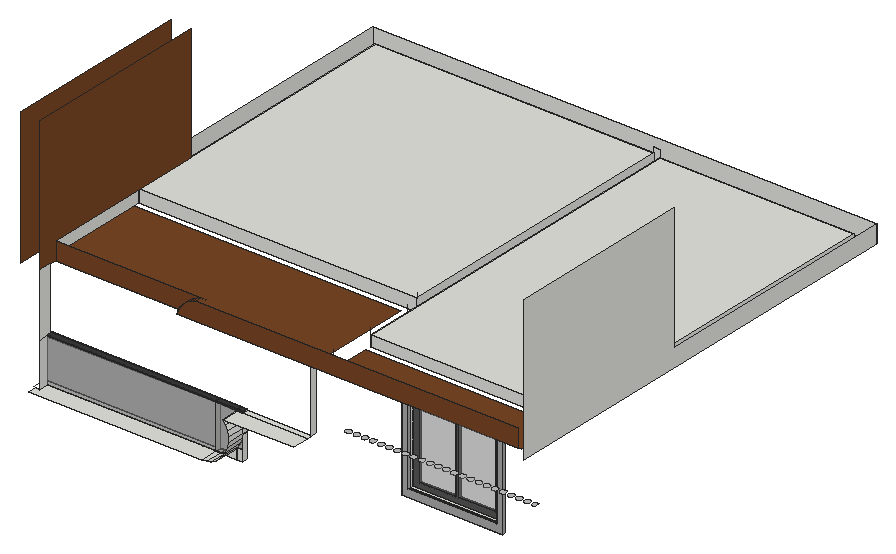
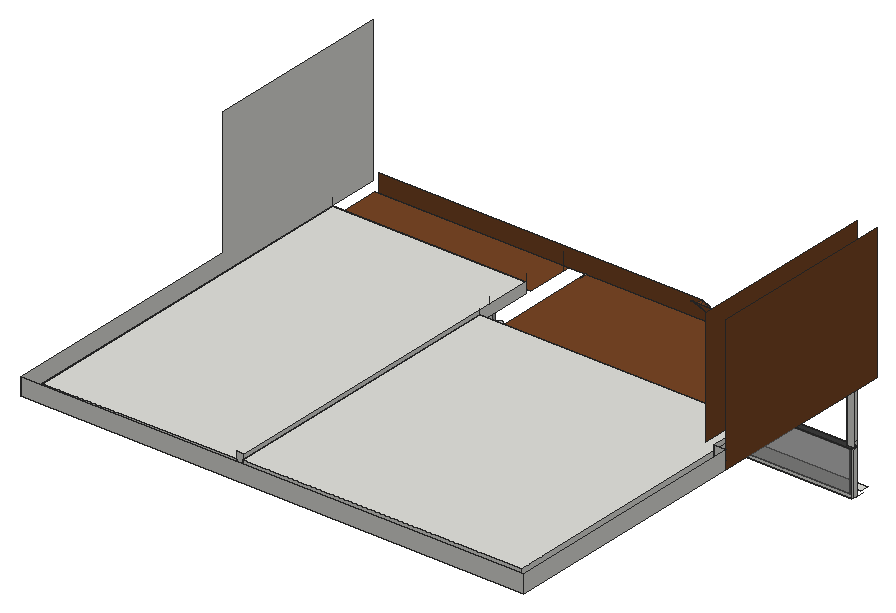
# SketchUp Ruby script. Lengths in millimetres.
U = 1.mm
M = Sketchup.active_model
def pt(a) = Geom::Point3d.new(a.map { |v| v * U })
def face(e, loops, mat)
  f = e.add_face(loops[0].map { |a| pt(a) })
  loops[1..].each { |l| e.add_face(l.map { |a| pt(a) }).erase! }
  f.material = f.back_material = mat if mat
  f
end
# faces: each face lists its corners as indices into pts; further lists are holes
def faces(e, pts, list, mat = nil) = list.each { |f| face(e, (f[0].is_a?(Array) ? f : [f]).map { |l| l.map { |i| pts[i] } }, mat) }
# xy, xz, yz: faces in a plane at the given z, y or x. An outline is a flat list of corners, or four numbers for a rectangle; further outlines are holes
def ring(l) = l.size == 4 ? [[l[0], l[1]], [l[2], l[1]], [l[2], l[3]], [l[0], l[3]]] : l.each_slice(2).to_a
def flat(e, list, mat, &to3) = list.each { |f| face(e, (f[0].is_a?(Array) ? f : [f]).map { |l| ring(l).map { |u, v| to3.(u, v) } }, mat) }
def xy(e, z, list, mat = nil) = flat(e, list, mat) { |x, y| [x, y, z] }
def xz(e, y, list, mat = nil) = flat(e, list, mat) { |x, z| [x, y, z] }
def yz(e, x, list, mat = nil) = flat(e, list, mat) { |y, z| [x, y, z] }
def lines(e, pts, list) = list.each { |a, b| e.add_line(pt(pts[a]), pt(pts[b])) }
# prism: a flat outline (further loops are holes) pulled along v
def prism(e, loops, v, mat = nil)
  f = face(e, loops, mat); d = Geom::Vector3d.new(v.map { |x| x * U })
  f.pushpull(f.normal.samedirection?(d) ? d.length : -d.length)
end
def box(e, o, s, mat = nil) = prism(e, [[o, [o[0] + s[0], o[1], o[2]], [o[0] + s[0], o[1] + s[1], o[2]], [o[0], o[1] + s[1], o[2]]]], [0, 0, s[2]], mat)
def at(x, y, z, deg = 0) = Geom::Transformation.translation(pt([x, y, z])) * Geom::Transformation.rotation(ORIGIN, Z_AXIS, deg.degrees)
def axes(o, x, y, z) = Geom::Transformation.new([*x, 0, *y, 0, *z, 0, *pt(o).to_a, 1])
def part(name) = M.definitions.add(name)
# library, detail: a bought-in or finely detailed component or shape, given as its bounding box
def library(name, o, s) = part(name).tap { |d| box(d.entities, o, s) }
def detail(e, o, s) = box(e.add_group.entities, o, s)
def put(e, d, t, mat = nil) = e.add_instance(d, t).tap { |i| i.material = mat if mat }
def group(e, t, mat = nil) = e.add_group.tap { |g| g.transformation = t; g.material = mat if mat }.entities
root = M.entities
M.materials.add("[Color M03]").color = [170, 170, 170]
M.materials.add("[Color M06]").color = [86, 86, 86]
M.materials.add("[Color M07]").color = [58, 58, 58]
M.materials.add("[Metal Corrugated Shiny]").color = [193, 193, 193]
M.materials.add("[Translucent Glass Gray]").color = [128, 128, 128]
M.materials["[Translucent Glass Gray]"].alpha = 0.5
M.materials.add("[Wood Veneer 01]").color = [120, 70, 37]
c1 = part("Group\#1")
xy(c1.entities,0,[[0,0,1355.7,60.3]],"[Color M06]")
xy(c1.entities,100.1,[[100.1,0,655.5,60.3],[696.9,0,1255.7,60.3]],"[Color M06]")
xy(c1.entities,1517.6,[[100.1,0,655.5,60.3],[696.9,0,1255.7,60.3]],"[Color M06]")
xy(c1.entities,1617.7,[[0,0,1355.7,60.3]],"[Color M06]")
xz(c1.entities,0,[[[0,0,1355.7,1617.7],[696.9,100.1,1255.7,1517.6],[100.1,100.1,655.5,1517.6]]],"[Color M06]")
xz(c1.entities,0,[[100.1,100.1,655.5,1517.6],[696.9,100.1,1255.7,1517.6]],"[Translucent Glass Gray]")
xz(c1.entities,60.3,[[[0,0,1355.7,1617.7],[696.9,100.1,1255.7,1517.6],[100.1,100.1,655.5,1517.6]]],"[Color M06]")
yz(c1.entities,0,[[0,0,60.3,1617.7]],"[Color M06]")
yz(c1.entities,100.1,[[0,100.1,60.3,1517.6]],"[Color M06]")
yz(c1.entities,655.5,[[0,100.1,60.3,1517.6]],"[Color M06]")
yz(c1.entities,696.9,[[0,100.1,60.3,1517.6]],"[Color M06]")
yz(c1.entities,1255.7,[[0,100.1,60.3,1517.6]],"[Color M06]")
yz(c1.entities,1355.7,[[0,0,60.3,1617.7]],"[Color M06]")
xy(root,4073.5,[[8130.9,1584.3,10586.8,1657.4]],"[Color M03]")
xy(root,4242.9,[[8275.8,1657.3,10434.8,1809.7]])
xy(root,4242.9,[[8275.8,1584.3,10434.8,1657.3]],"[Color M03]")
xy(root,4272.1,[[374.7,0,4556.2,0,4556.2,424.6,479.5,424.6,479.5,209.6,374.7,209.6],[308.1,424.6,4556.2,555.6],[4556.2,424.6,5081.7,555.6],[5081.7,424.6,5214.2,555.6]])
xy(root,5334,[[5080.9,0,6787.6,424.6],[5080.9,424.6,5081.7,555.6],[5214.2,424.6,6787.6,555.6]])
xy(root,5334,[[308.1,424.6,4556.2,555.6],[4556.2,424.6,5080.9,555.6],[5081.7,424.6,5214.2,555.6]],"[Color M07]")
xy(root,5372.1,[[308.1,424.6,479.5,514.4]])
xy(root,5372.1,[[479.5,424.6,4556.2,424.6,4556.2,555.6,308.1,555.6,308.1,514.4,479.5,514.4],[4556.2,424.6,5080.9,555.6],[5081.7,424.6,5214.2,555.6]],"[Color M07]")
xy(root,5423.4,[[7323,932.9,7339.9,934.9,7355.7,941.2,7369.3,951.3,7379.8,964.7,7386.5,980.3,7389,997.1,7387,1014,7380.7,1029.8,7370.6,1043.4,7357.2,1053.9,7341.6,1060.6,7324.8,1063.1,7307.9,1061.1,7292.1,1054.8,7278.5,1044.7,7268,1031.3,7261.3,1015.7,7258.8,998.9,7260.8,982,7267.1,966.2,7277.2,952.6,7290.6,942.1,7306.2,935.4],[7519.8,932.9,7536.7,934.9,7552.5,941.2,7566.1,951.3,7576.7,964.7,7583.4,980.3,7585.8,997.1,7583.8,1014,7577.6,1029.8,7567.4,1043.4,7554.1,1053.9,7538.5,1060.6,7521.6,1063.1,7504.8,1061.1,7489,1054.8,7475.4,1044.7,7464.8,1031.3,7458.1,1015.7,7455.7,998.9,7457.6,982,7463.9,966.2,7474.1,952.6,7487.4,942.1,7503,935.4],[7716.7,932.9,7733.6,934.9,7749.4,941.2,7763,951.3,7773.5,964.7,7780.2,980.3,7782.7,997.1,7780.7,1014,7774.4,1029.8,7764.3,1043.4,7750.9,1053.9,7735.3,1060.6,7718.5,1063.1,7701.6,1061.1,7685.8,1054.8,7672.2,1044.7,7661.7,1031.3,7655,1015.7,7652.5,998.9,7654.5,982,7660.8,966.2,7670.9,952.6,7684.3,942.1,7699.9,935.4],[7913.5,932.9,7930.4,934.9,7946.2,941.2,7959.8,951.3,7970.4,964.7,7977.1,980.3,7979.5,997.1,7977.5,1014,7971.3,1029.8,7961.1,1043.4,7947.8,1053.9,7932.2,1060.6,7915.3,1063.1,7898.5,1061.1,7882.7,1054.8,7869.1,1044.7,7858.5,1031.3,7851.8,1015.7,7849.4,998.9,7851.3,982,7857.6,966.2,7867.8,952.6,7881.1,942.1,7896.7,935.4],[8110.4,932.9,8127.3,934.9,8143.1,941.2,8156.7,951.3,8167.2,964.7,8173.9,980.3,8176.4,997.1,8174.4,1014,8168.1,1029.8,8158,1043.4,8144.6,1053.9,8129,1060.6,8112.2,1063.1,8095.3,1061.1,8079.5,1054.8,8065.9,1044.7,8055.4,1031.3,8048.7,1015.7,8046.2,998.9,8048.2,982,8054.5,966.2,8064.6,952.6,8078,942.1,8093.6,935.4],
  [8307.2,932.9,8324.1,934.9,8339.9,941.2,8353.5,951.3,8364.1,964.7,8370.8,980.3,8373.2,997.1,8371.2,1014,8365,1029.8,8354.8,1043.4,8341.5,1053.9,8325.9,1060.6,8309,1063.1,8292.2,1061.1,8276.4,1054.8,8262.8,1044.7,8252.2,1031.3,8245.5,1015.7,8243.1,998.9,8245,982,8251.3,966.2,8261.5,952.6,8274.8,942.1,8290.4,935.4],[8504.1,932.9,8521,934.9,8536.8,941.2,8550.4,951.3,8560.9,964.7,8567.6,980.3,8570.1,997.1,8568.1,1014,8561.8,1029.8,8551.7,1043.4,8538.3,1053.9,8522.7,1060.6,8505.9,1063.1,8489,1061.1,8473.2,1054.8,8459.6,1044.7,8449.1,1031.3,8442.4,1015.7,8439.9,998.9,8441.9,982,8448.2,966.2,8458.3,952.6,8471.7,942.1,8487.3,935.4],[8700.9,932.9,8717.8,934.9,8733.6,941.2,8747.2,951.3,8757.8,964.7,8764.5,980.3,8766.9,997.1,8764.9,1014,8758.7,1029.8,8748.5,1043.4,8735.2,1053.9,8719.6,1060.6,8702.7,1063.1,8685.9,1061.1,8670.1,1054.8,8656.5,1044.7,8645.9,1031.3,8639.2,1015.7,8636.8,998.9,8638.7,982,8645,966.2,8655.2,952.6,8668.5,942.1,8684.1,935.4],[8897.8,932.9,8914.7,934.9,8930.5,941.2,8944.1,951.3,8954.6,964.7,8961.3,980.3,8963.8,997.1,8961.8,1014,8955.5,1029.8,8945.4,1043.4,8932,1053.9,8916.4,1060.6,8899.6,1063.1,8882.7,1061.1,8866.9,1054.8,8853.3,1044.7,8842.8,1031.3,8836.1,1015.7,8833.6,998.9,8835.6,982,8841.9,966.2,8852,952.6,8865.4,942.1,8881,935.4],[9094.6,932.9,9111.5,934.9,9127.3,941.2,9140.9,951.3,9151.5,964.7,9158.2,980.3,9160.6,997.1,9158.6,1014,9152.4,1029.8,9142.2,1043.4,9128.9,1053.9,9113.3,1060.6,9096.4,1063.1,9079.6,1061.1,9063.8,1054.8,9050.2,1044.7,9039.6,1031.3,9032.9,1015.7,9030.5,998.9,9032.4,982,9038.7,966.2,9048.9,952.6,9062.2,942.1,9077.8,935.4],
  [9291.5,932.9,9308.4,934.9,9324.2,941.2,9337.8,951.3,9348.3,964.7,9355,980.3,9357.5,997.1,9355.5,1014,9349.2,1029.8,9339.1,1043.4,9325.7,1053.9,9310.1,1060.6,9293.3,1063.1,9276.4,1061.1,9260.6,1054.8,9247,1044.7,9236.5,1031.3,9229.8,1015.7,9227.3,998.9,9229.3,982,9235.6,966.2,9245.7,952.6,9259.1,942.1,9274.7,935.4],[9488.3,932.9,9505.2,934.9,9521,941.2,9534.6,951.3,9545.2,964.7,9551.9,980.3,9554.3,997.1,9552.3,1014,9546.1,1029.8,9535.9,1043.4,9522.6,1053.9,9507,1060.6,9490.1,1063.1,9473.3,1061.1,9457.5,1054.8,9443.9,1044.7,9433.3,1031.3,9426.6,1015.7,9424.2,998.9,9426.1,982,9432.4,966.2,9442.6,952.6,9455.9,942.1,9471.5,935.4],[9685.2,932.9,9702.1,934.9,9717.9,941.2,9731.5,951.3,9742,964.7,9748.7,980.3,9751.2,997.1,9749.2,1014,9742.9,1029.8,9732.8,1043.4,9719.4,1053.9,9703.8,1060.6,9687,1063.1,9670.1,1061.1,9654.3,1054.8,9640.7,1044.7,9630.2,1031.3,9623.5,1015.7,9621,998.9,9623,982,9629.3,966.2,9639.4,952.6,9652.8,942.1,9668.4,935.4],[9882,932.9,9898.9,934.9,9914.7,941.2,9928.3,951.3,9938.9,964.7,9945.6,980.3,9948,997.1,9946,1014,9939.8,1029.8,9929.6,1043.4,9916.3,1053.9,9900.7,1060.6,9883.8,1063.1,9867,1061.1,9851.2,1054.8,9837.6,1044.7,9827,1031.3,9820.3,1015.7,9817.9,998.9,9819.8,982,9826.1,966.2,9836.3,952.6,9849.6,942.1,9865.2,935.4],[10078.9,932.9,10095.8,934.9,10111.6,941.2,10125.2,951.3,10135.7,964.7,10142.4,980.3,10144.9,997.1,10142.9,1014,10136.6,1029.8,10126.5,1043.4,10113.1,1053.9,10097.5,1060.6,10080.7,1063.1,10063.8,1061.1,10048,1054.8,10034.4,1044.7,10023.9,1031.3,10017.2,1015.7,10014.7,998.9,10016.7,982,10023,966.2,10033.1,952.6,10046.5,942.1,10062.1,935.4],
  [10275.7,932.9,10292.6,934.9,10308.4,941.2,10322,951.3,10332.6,964.7,10339.3,980.3,10341.7,997.1,10339.7,1014,10333.5,1029.8,10323.3,1043.4,10310,1053.9,10294.4,1060.6,10277.5,1063.1,10260.7,1061.1,10244.9,1054.8,10231.3,1044.7,10220.7,1031.3,10214,1015.7,10211.6,998.9,10213.5,982,10219.8,966.2,10230,952.6,10243.3,942.1,10258.9,935.4],[10472.6,932.9,10489.5,934.9,10505.3,941.2,10518.9,951.3,10529.4,964.7,10536.1,980.3,10538.6,997.1,10536.6,1014,10530.3,1029.8,10520.2,1043.4,10506.8,1053.9,10491.2,1060.6,10474.4,1063.1,10457.5,1061.1,10441.7,1054.8,10428.1,1044.7,10417.6,1031.3,10410.9,1015.7,10408.4,998.9,10410.4,982,10416.7,966.2,10426.8,952.6,10440.2,942.1,10455.8,935.4],[10669.4,932.9,10686.3,934.9,10702.1,941.2,10715.7,951.3,10726.3,964.7,10733,980.3,10735.4,997.1,10733.4,1014,10727.2,1029.8,10717,1043.4,10703.7,1053.9,10688.1,1060.6,10671.2,1063.1,10654.4,1061.1,10638.6,1054.8,10625,1044.7,10614.4,1031.3,10607.7,1015.7,10605.3,998.9,10607.2,982,10613.5,966.2,10623.7,952.6,10637,942.1,10652.6,935.4],[10866.3,932.9,10883.2,934.9,10899,941.2,10912.6,951.3,10923.1,964.7,10929.8,980.3,10932.3,997.1,10930.3,1014,10924,1029.8,10913.9,1043.4,10900.5,1053.9,10884.9,1060.6,10868.1,1063.1,10851.2,1061.1,10835.4,1054.8,10821.8,1044.7,10811.3,1031.3,10804.6,1015.7,10802.1,998.9,10804.1,982,10810.4,966.2,10820.5,952.6,10833.9,942.1,10849.5,935.4],[11063.1,932.9,11080,934.9,11095.8,941.2,11109.4,951.3,11120,964.7,11126.7,980.3,11129.1,997.1,11127.1,1014,11120.9,1029.8,11110.7,1043.4,11097.4,1053.9,11081.8,1060.6,11064.9,1063.1,11048.1,1061.1,11032.3,1054.8,11018.7,1044.7,11008.1,1031.3,11001.4,1015.7,10999,998.9,11000.9,982,11007.2,966.2,11017.4,952.6,11030.7,942.1,11046.3,935.4],
  [11260,932.9,11276.9,934.9,11292.7,941.2,11306.3,951.3,11316.8,964.7,11323.5,980.3,11326,997.1,11324,1014,11317.7,1029.8,11307.6,1043.4,11294.2,1053.9,11278.6,1060.6,11261.8,1063.1,11244.9,1061.1,11229.1,1054.8,11215.5,1044.7,11205,1031.3,11198.3,1015.7,11195.8,998.9,11197.8,982,11204.1,966.2,11214.2,952.6,11227.6,942.1,11243.2,935.4],[11456.8,932.9,11473.7,934.9,11489.5,941.2,11503.1,951.3,11513.7,964.7,11520.4,980.3,11522.8,997.1,11520.8,1014,11514.6,1029.8,11504.4,1043.4,11491.1,1053.9,11475.5,1060.6,11458.6,1063.1,11441.8,1061.1,11426,1054.8,11412.4,1044.7,11401.8,1031.3,11395.1,1015.7,11392.7,998.9,11394.6,982,11400.9,966.2,11411.1,952.6,11424.4,942.1,11440,935.4],[11653.7,932.9,11670.6,934.9,11686.4,941.2,11700,951.3,11710.5,964.7,11717.2,980.3,11719.7,997.1,11717.7,1014,11711.4,1029.8,11701.3,1043.4,11687.9,1053.9,11672.3,1060.6,11655.5,1063.1,11638.6,1061.1,11622.8,1054.8,11609.2,1044.7,11598.7,1031.3,11592,1015.7,11589.5,998.9,11591.5,982,11597.8,966.2,11607.9,952.6,11621.3,942.1,11636.9,935.4],[11850.5,932.9,11867.4,934.9,11883.2,941.2,11890.5,946.6,11890.5,1049.4,11884.8,1053.9,11869.2,1060.6,11852.3,1063.1,11835.5,1061.1,11819.7,1054.8,11806.1,1044.7,11795.5,1031.3,11788.8,1015.7,11786.4,998.9,11788.3,982,11794.6,966.2,11804.8,952.6,11818.1,942.1,11833.7,935.4]],"[Metal Corrugated Shiny]")
xy(root,6383.1,[[2137.7,3257.5,4426,3410]])
xy(root,6401.9,[[8275.8,1657.3,10434.8,1809.7]])
xy(root,6401.9,[[8275.8,1584.3,10434.8,1657.3]],"[Color M03]")
xy(root,6529.3,[[8130.9,1584.3,10586.8,1657.4]],"[Color M03]")
xy(root,6858,[[308.1,514.4,479.5,687.4]])
xy(root,6858,[[3547.8,514.4,3547.8,687.4,308.1,687.4,308.1,3257.6,6787.6,3257.6,6787.6,514.4],[7199.4,514.4,11890.5,1657.4]],"[Wood Veneer 01]")
xy(root,7112,[[7199.4,1809.8,11890.5,10572.8]])
xy(root,7162.8,[[308.1,3410,7047,10572.8]])
xz(root,424.6,[[308.1,4272.1,479.5,5334],[4556.2,4272.1,5081.7,4272.1,5081.7,4533,5002.2,4445.4,4904.8,4371.6,4795.5,4317,4677.9,4283.4],[5081.7,4272.1,5214.2,4533],[5081.7,4533,5214.2,4533,5214.2,5332.7,5081.7,5332.7,5145.9,5230.5,5190.6,5116.7,5213.7,4996.7,5214.2,4874.4,5192.2,4754.2,5148.4,4640.1,5084.4,4536],[5081.7,5332.7,5081.7,5334,5080.9,5334],
  [5081.7,5332.7,5214.2,5334],[308.1,5334,479.5,5372.1]])
xz(root,424.6,[[479.5,5334,4556.2,5372.1],[4556.2,5334,5080.9,5372.1],[5081.7,5334,5214.2,5372.1]],"[Color M07]")
xz(root,424.6,[[479.5,4272.1,4556.2,5334],[4556.2,4272.1,4677.9,4283.4,4795.5,4317,4904.8,4371.6,5002.2,4445.4,5081.7,4533,5081.7,5332.7,5080.9,5334,4556.2,5334],[5081.7,4533,5214.2,5332.7]],"[Translucent Glass Gray]")
xz(root,514.4,[[308.1,5372.1,479.5,6858]])
xz(root,514.4,[[3547.8,6858,11814.3,6858,11814.3,7289.8,4112.5,7289.8,4048.9,7286.3,3986.1,7276,3924.8,7258.9,3865.8,7235.3,3809.6,7205.3,3757,7169.5,3708.7,7128.1,3665.1,7081.8,3626.8,7031,3594.2,6976.3,3567.8,6918.4]],"[Wood Veneer 01]")
xz(root,555.6,[[4556.2,4272.1,4677.9,4283.4,4795.5,4317,4904.8,4371.6,5002.2,4445.4,5081.7,4533,5081.7,4272.1],[5081.7,4272.1,5214.2,4533],[5081.7,4533,5084.4,4536,5148.4,4640.1,5192.2,4754.2,5214.2,4874.4,5213.7,4996.7,5190.6,5116.7,5145.9,5230.5,5081.7,5332.7,5214.2,5332.7,5214.2,4533],[5081.7,5332.7,5080.9,5334,5081.7,5334],[5081.7,5332.7,5214.2,5334]])
xz(root,555.6,[[308.1,5334,4556.2,5372.1],[4556.2,5334,5080.9,5372.1],[5081.7,5334,5214.2,5372.1]],"[Color M07]")
xz(root,555.6,[[308.1,4272.1,4556.2,5334],[4556.2,4272.1,4556.2,5334,5080.9,5334,5081.7,5332.7,5081.7,4533,5002.2,4445.4,4904.8,4371.6,4795.5,4317,4677.9,4283.4],[5081.7,4533,5214.2,5332.7]],"[Translucent Glass Gray]")
xz(root,687.4,[[308.1,6858,479.5,7289.8]])
xz(root,687.4,[[479.5,6858,3547.8,6858,3567.8,6918.4,3594.2,6976.3,3626.8,7031,3665.1,7081.8,3708.7,7128.1,3757,7169.5,3809.6,7205.3,3865.8,7235.3,3924.8,7258.9,3986.1,7276,4048.9,7286.3,4112.5,7289.8,479.5,7289.8]],"[Wood Veneer 01]")
xz(root,1584.3,[[[8130.9,4073.5,10586.8,6529.3],[8275.8,4242.9,10434.8,6401.9]]],"[Color M03]")
xz(root,1809.8,[[7199.4,6858,11890.5,7112]])
xz(root,3410,[[308.1,6858,7047,7162.8]])
xz(root,4760.9,[[3.3,6858,308.1,7289.8]])
xz(root,10572.8,[[308.1,6858,7047,7162.8],[7047,6858,7199.4,7289.8],[7199.4,6858,11890.5,7112]])
xz(root,10877.6,[[3.3,6858,12195.3,7289.8]])
yz(root,3.3,[[4760.9,6858,10877.6,7289.8]])
yz(root,3.3,[[209.6,6858,4760.9,10119.6]],"[Wood Veneer 01]")
yz(root,308.1,[[424.6,4272.1,514.4,5334],[514.4,4272.1,555.6,5334],[687.4,6858,3410,6858,3410,7162.8,4181.5,7162.8,4181.5,7289.8,687.4,7289.8],[3410,6858,4760.9,7162.8],[4760.9,6858,10572.8,7162.8],
  [4181.5,7162.8,4760.9,7289.8]])
yz(root,308.1,[[424.6,5334,514.4,5372.1],[514.4,5334,555.6,5372.1]],"[Color M07]")
yz(root,479.5,[[209.6,4272.1,424.6,5334],[209.6,5334,424.6,5334,424.6,5372.1,514.4,5372.1,514.4,6858,209.6,6858]])
yz(root,479.5,[[209.6,6858,687.4,6858,687.4,7289.8,4760.9,7289.8,4760.9,10096.5,209.6,10096.5]],"[Wood Veneer 01]")
yz(root,4556.2,[[424.6,4272.1,555.6,5334]])
yz(root,4556.2,[[424.6,5334,555.6,5372.1]],"[Color M07]")
yz(root,5080.9,[[424.6,5334,555.6,5372.1]],"[Color M07]")
yz(root,5081.7,[[424.6,4272.1,555.6,5334]])
yz(root,5081.7,[[424.6,5334,555.6,5372.1]],"[Color M07]")
yz(root,5214.2,[[424.6,4272.1,555.6,4874.4],[424.6,4874.4,555.6,5334]])
yz(root,5214.2,[[424.6,5334,555.6,5372.1]],"[Color M07]")
yz(root,6787.6,[[514.4,5334,687.4,6858]])
yz(root,7047,[[3410,6858,10572.8,7162.8]])
yz(root,7199.4,[[1809.8,6858,10572.8,7112]])
yz(root,8130.9,[[1584.3,4073.5,1657.4,6529.3]],"[Color M03]")
yz(root,8275.8,[[1657.3,4242.9,1809.7,6401.9]])
yz(root,8275.8,[[1584.3,4242.9,1657.3,6401.9]],"[Color M03]")
yz(root,10434.8,[[1657.3,4242.9,1809.7,6401.9]])
yz(root,10434.8,[[1584.3,4242.9,1657.3,6401.9]],"[Color M03]")
yz(root,10586.8,[[1584.3,4073.5,1657.4,6529.3]],"[Color M03]")
yz(root,11890.5,[[1809.8,6858,10572.8,7112]])
yz(root,12195.3,[[209.6,6858,10877.6,6858,10877.6,7289.8,4760.9,7289.8,4760.9,10337.8,209.6,10337.8]])
p = [[8130.9,1657.4,6529.3],[10586.8,1657.4,6529.3],[10586.8,1657.4,4073.5],[8130.9,1657.4,4073.5],[8275.8,1657.3,4242.9],[10434.8,1657.3,4242.9],
  [10434.8,1657.3,6401.9],[8275.8,1657.3,6401.9],[4556.2,424.6,4272.1],[4556.2,0,4272.1],[4677.9,0,4283.4],[4677.9,424.6,4283.4],
  [4677.9,555.6,4283.4],[4556.2,555.6,4272.1],[4795.5,0,4317],[4795.5,424.6,4317],[4795.5,555.6,4317],[4904.8,0,4371.6],
  [4904.8,424.6,4371.6],[4904.8,555.6,4371.6],[5002.2,0,4445.4],[5002.2,424.6,4445.4],[5002.2,555.6,4445.4],[5084.4,0,4536],
  [5084.4,424.6,4536],[5081.7,424.6,4533],[5084.4,555.6,4536],[5081.7,555.6,4533],[5148.4,0,4640.1],[5148.4,424.6,4640.1],
  [5148.4,555.6,4640.1],[5192.2,0,4754.2],[5192.2,424.6,4754.2],[5192.2,555.6,4754.2],[5214.2,0,4874.4],[5214.2,424.6,4874.4],
  [5214.2,555.6,4874.4],[5213.7,0,4996.7],[5213.7,424.6,4996.7],[5213.7,555.6,4996.7],[5190.6,0,5116.7],[5190.6,424.6,5116.7],
  [5190.6,555.6,5116.7],[5145.9,0,5230.5],[5145.9,424.6,5230.5],[5145.9,555.6,5230.5],[5080.9,0,5334],[5080.9,424.6,5334],
  [5081.7,424.6,5332.7],[5080.9,555.6,5334],[5081.7,555.6,5332.7],[3567.8,687.4,6918.4],[3547.8,687.4,6858],[3547.8,514.4,6858],
  [3567.8,514.4,6918.4],[3594.2,687.4,6976.3],[3594.2,514.4,6976.3],[3626.8,687.4,7031],[3626.8,514.4,7031],[3665.1,687.4,7081.8],
  [3665.1,514.4,7081.8],[3708.7,687.4,7128.1],[3708.7,514.4,7128.1],[3757,687.4,7169.5],[3757,514.4,7169.5],[3809.6,687.4,7205.3],
  [3809.6,514.4,7205.3],[3865.8,687.4,7235.3],[3865.8,514.4,7235.3],[3924.8,687.4,7258.9],[3924.8,514.4,7258.9],[3986.1,687.4,7276],
  [3986.1,514.4,7276],[7199.4,687.4,7289.8],[7199.4,687.4,6858],[308.1,209.6,4272.1],[308.1,424.6,4272.1],[7199.4,2931.6,7289.8],
  [7199.4,2931.6,7112],[11890.5,1809.8,7112],[11890.5,1809.8,7289.8],[7199.4,1809.8,7112],[7199.4,1809.8,7289.8],[7047,3410,7162.8],
  [7047,3410,7289.8]]
faces(root,p,[[[0,1,2,3],[4,5,6,7]],[8,9,10,11],[8,11,12,13],[11,10,14,15],[11,15,16,12],[15,14,17,18],[15,18,19,16],[18,17,20,21],
  [18,21,22,19],[21,20,23,24,25],[21,25,24,26,27,22],[24,23,28,29],[24,29,30,26],[29,28,31,32],[29,32,33,30],[32,31,34,35],
  [32,35,36,33],[35,34,37,38],[35,38,39,36],[38,37,40,41],[38,41,42,39],[41,40,43,44],[41,44,45,42],[44,43,46,47,48],
  [44,48,47,49,50,45]])
faces(root,p,[[51,52,53,54],[55,51,54,56],[57,55,56,58],[59,57,58,60],[61,59,60,62],[63,61,62,64],[65,63,64,66],[67,65,66,68],
  [69,67,68,70],[71,69,70,72]],"[Wood Veneer 01]")
lines(root,p,[[73,74],[75,76],[77,78],[79,80],[81,82],[83,84]])
put(root,c1,axes([8275.8,1749.4,4242.9],[1.59251,0,0],[0,0.84,0],[0,0,1.33464]))
